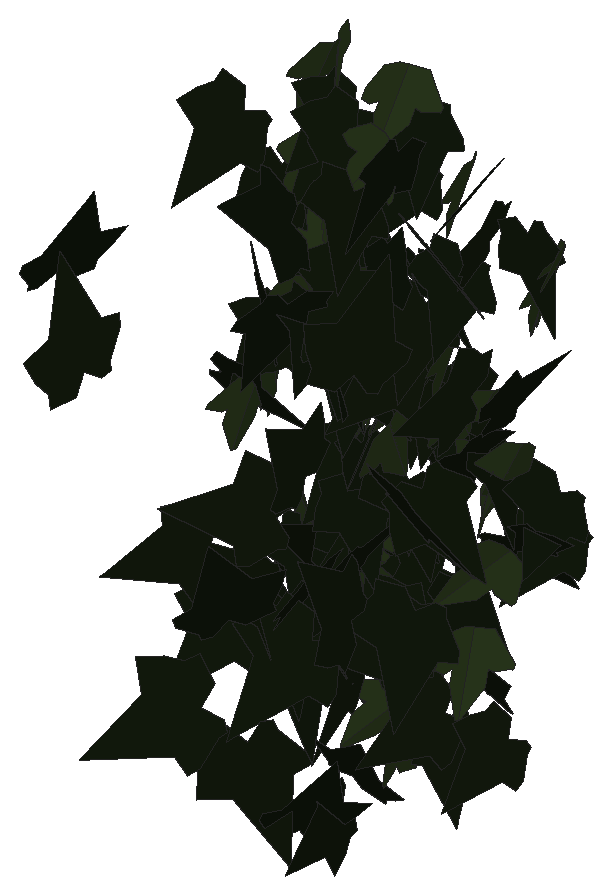
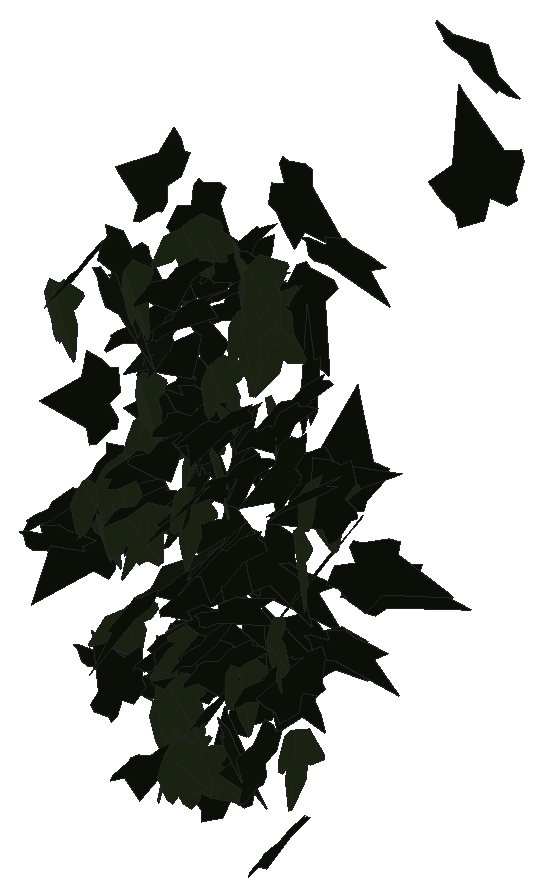
# SketchUp Ruby script. Lengths in inches.
U = 1.inch
M = Sketchup.active_model
def pt(a) = Geom::Point3d.new(a.map { |v| v * U })
def face(e, loops, mat)
  f = e.add_face(loops[0].map { |a| pt(a) })
  loops[1..].each { |l| e.add_face(l.map { |a| pt(a) }).erase! }
  f.material = f.back_material = mat if mat
  f
end
# faces: each face lists its corners as indices into pts; further lists are holes
def faces(e, pts, list, mat = nil) = list.each { |f| face(e, (f[0].is_a?(Array) ? f : [f]).map { |l| l.map { |i| pts[i] } }, mat) }
# xy, xz, yz: faces in a plane at the given z, y or x. An outline is a flat list of corners, or four numbers for a rectangle; further outlines are holes
def ring(l) = l.size == 4 ? [[l[0], l[1]], [l[2], l[1]], [l[2], l[3]], [l[0], l[3]]] : l.each_slice(2).to_a
def flat(e, list, mat, &to3) = list.each { |f| face(e, (f[0].is_a?(Array) ? f : [f]).map { |l| ring(l).map { |u, v| to3.(u, v) } }, mat) }
def xy(e, z, list, mat = nil) = flat(e, list, mat) { |x, y| [x, y, z] }
def xz(e, y, list, mat = nil) = flat(e, list, mat) { |x, z| [x, y, z] }
def yz(e, x, list, mat = nil) = flat(e, list, mat) { |y, z| [x, y, z] }
def lines(e, pts, list) = list.each { |a, b| e.add_line(pt(pts[a]), pt(pts[b])) }
# prism: a flat outline (further loops are holes) pulled along v
def prism(e, loops, v, mat = nil)
  f = face(e, loops, mat); d = Geom::Vector3d.new(v.map { |x| x * U })
  f.pushpull(f.normal.samedirection?(d) ? d.length : -d.length)
end
def box(e, o, s, mat = nil) = prism(e, [[o, [o[0] + s[0], o[1], o[2]], [o[0] + s[0], o[1] + s[1], o[2]], [o[0], o[1] + s[1], o[2]]]], [0, 0, s[2]], mat)
def at(x, y, z, deg = 0) = Geom::Transformation.translation(pt([x, y, z])) * Geom::Transformation.rotation(ORIGIN, Z_AXIS, deg.degrees)
def axes(o, x, y, z) = Geom::Transformation.new([*x, 0, *y, 0, *z, 0, *pt(o).to_a, 1])
def part(name) = M.definitions.add(name)
# library, detail: a bought-in or finely detailed component or shape, given as its bounding box
def library(name, o, s) = part(name).tap { |d| box(d.entities, o, s) }
def detail(e, o, s) = box(e.add_group.entities, o, s)
def put(e, d, t, mat = nil) = e.add_instance(d, t).tap { |i| i.material = mat if mat }
def group(e, t, mat = nil) = e.add_group.tap { |g| g.transformation = t; g.material = mat if mat }.entities
root = M.entities
M.materials.add("efeu1").color = [18, 25, 13]
M.materials.add("efeu2").color = [43, 57, 29]
c1 = part("ivyleaf_9")
p = [[1.54,2.16,1.25],[1.36,2.04,1.19],[-0.21,0.99,0.68],[-0.71,1.11,0.82],[-0.85,0.86,0.67],[-0.8,0.17,0.21],
  [-0.9,-0.01,0.1],[-0.67,-0.16,-0.02],[-0.08,-0.08,-0.05],[-0.03,-0.6,-0.4],[0.65,-0.88,-0.66],[0.83,-0.6,-0.49],
  [1.29,-0.42,-0.43],[1.8125,-0.07,-0.26],[1.21,0.44,0.15]]
faces(c1.entities,p,[[0,1,2,3,4,5,6,7,8,9,10,11,12,13,14]],"efeu1")
c2 = part("ivyleaf_10")
p = [[0,0.5,-0.03],[-0.0625,2.02,-0.43],[-0.19,2.01,-0.46],[-0.54,1.05,-0.29],[-0.52,0.625,-0.18],[-0.83,0.76,-0.28],
  [-1.16,0.64,-0.33],[-1.15,0.33,-0.24],[-0.77,-0.39,0.02],[-0.3,-0.51,0.16],[0.04,-0.48,0.23],[-0.02,2.01,-0.4375],
  [-0.06,2.01,-0.43],[0.04,-0.49,0.23],[0.67,-0.49,0.14],[1.38,0.36,-0.2],[1.375,0.51,-0.24],[0.81,0.65,-0.19],
  [0.62,0.59,-0.15],[0.6,1.09,-0.28],[0.5,1.23,-0.31]]
faces(c2.entities,p,[[0,1,2,3,4,5,6,7,8,9,10],[11,12,0,13,14,15,16,17,18,19,20]],"efeu2")
put(root,c1,axes([586.75,103.9375,300.07],[-1.43697,0.25356,-0.39672],[-0.40228,0.00084,1.45765],[0.24464,1.49073,0.06665]))
put(root,c1,axes([580.63,110.38,299],[0.80023,1.1061,0.65598],[-0.38497,-0.53115,1.36522],[1.22701,-0.88802,0.00051]))
put(root,c1,axes([584.13,113.52,281.39],[-1.16182,-0.52267,0.7875],[-0.71796,-0.32355,-1.27397],[0.61471,-1.36576,0.00044]))
put(root,c1,axes([585.37,113.77,285.38],[0.86867,0.58087,1.00057],[-0.81836,-0.57596,1.04485],[0.81783,-1.19332,-0.01725]))
put(root,c1,axes([589.24,113.0625,292.68],[-0.47842,0.80905,1.0484],[-0.56196,0.88534,-0.93966],[-1.19913,-0.7377,0.02208]))
put(root,c1,axes([585.23,115.08,279.55],[-0.59414,-0.71943,-1.18347],[0.79414,0.87809,-0.93247],[1.13469,-0.99125,0.03293]))
put(root,c1,axes([590.02,114.63,286.51],[-0.82384,0.13634,-1.1871],[-1.19412,-0.04146,0.82395],[0.04349,1.44437,0.1357]))
put(root,c1,axes([586.875,115.93,276.61],[0.99318,0.88272,0.41487],[-0.31395,-0.27126,1.32874],[0.92344,-1.0416,0.00555]))
put(root,c1,axes([587.57,117.14,276.97],[0.02429,-0.43729,-1.21261],[0.81544,-0.93412,0.35319],[-0.99836,-0.7736,0.25898]))
put(root,c1,axes([584.55,117.18,287.53],[-0.67759,-0.1305,1.15622],[-1.11265,-0.31875,-0.68804],[0.34039,-1.30168,0.05257]))
put(root,c1,axes([585.93,116.39,300.05],[-0.34419,0.20999,-1.38623],[-1.34021,-0.46852,0.26179],[-0.4118,1.34929,0.30664]))
put(root,c1,axes([585.91,117.46,282.89],[-1.34941,-0.66672,0.05597],[-0.05103,-0.02307,-1.50513],[0.66711,-1.35037,-0.00192]))
put(root,c1,axes([581.37,117.58,285.15],[-0.15915,-0.22662,-1.32348],[-0.57593,-1.19241,0.27343],[-1.21296,0.59591,0.04382]))
put(root,c1,axes([585.25,117.13,296.08],[-0.01644,1.00641,-0.92606],[0.05511,-0.92488,-1.00611],[-1.36653,-0.04941,-0.02943]))
put(root,c1,axes([588.62,116.69,295.01],[-0.73567,-0.51703,1.10661],[0.95074,0.5686,0.89771],[-0.7668,1.20103,0.05138]))
put(root,c1,axes([583.59,118.55,283.49],[0.59643,-1.16339,-0.67837],[0.3067,-0.60509,1.30737],[-1.31134,-0.67066,-0.00278]))
put(root,c1,axes([589.88,118.38,284.96],[-0.31241,-1.44345,0.12125],[0.04691,-0.13405,-1.47502],[1.44778,-0.30714,0.07396]))
put(root,c1,axes([585.31,118.65,294.98],[-0.05503,-1.06245,0.60991],[0.01412,-0.61103,-1.06314],[1.22499,-0.04068,0.03965]))
put(root,c1,axes([589.23,118.1,289.51],[1.02422,-0.74101,0.78859],[0.65085,-0.44562,-1.26405],[0.86451,1.21339,0.01737]))
put(root,c1,axes([585.54,118.18,284.93],[-0.65386,0.991,-0.59397],[0.25392,-0.54255,-1.18473],[-1.12712,-0.69712,0.07767]))
put(root,c1,axes([590.31,118.61,299.625],[0.69046,-0.84039,0.77859],[0.58148,-0.52618,-1.08361],[0.98709,0.89781,0.09373]))
put(root,c1,axes([581.75,118.77,282.01],[-1.28329,-0.42191,0.02426],[-0.0225,-0.00923,-1.35086],[0.42201,-1.28348,0.00174]))
put(root,c1,axes([591.98,118.76,294.17],[-1.15821,0.86921,0.23179],[-0.22706,0.08317,-1.44646],[-0.87046,-1.17824,0.06889]))
put(root,c1,axes([586.01,120.07,296.42],[-0.66991,-1.09414,0.35514],[-0.14803,-0.32555,-1.28224],[1.14076,-0.68478,0.04216]))
put(root,c1,axes([581.82,120.22,293.23],[-0.19244,0.08248,1.46618],[0.29567,-1.44626,0.12017],[1.43843,0.30831,0.17145]))
put(root,c1,axes([588.39,120.34,282.33],[-0.67766,-0.26939,1.09771],[-0.95641,-0.54541,-0.72428],[0.60235,-1.16907,0.08495]))
put(root,c1,axes([580.71,120.23,300.82],[-1.32776,-0.38705,-0.13705],[0.13425,0.02916,-1.38299],[0.38803,-1.33449,0.00953]))
put(root,c1,axes([585.42,120.58,299.11],[-0.10894,-1.25254,0.23472],[-0.01925,-0.23393,-1.25727],[1.2742,-0.11062,0.00108]))
put(root,c2,axes([584.23,119.79,295.39],[-1.08822,-0.53728,-0.16161],[0.13842,0.08466,-1.21354],[0.54372,-1.0969,-0.0145]))
put(root,c1,axes([589.26,119.76,289],[0.29444,-0.93222,-0.91034],[-0.03406,0.92747,-0.96078],[1.30253,0.23498,0.18066]))
put(root,c1,axes([585.85,119.1,284.73],[-0.18735,1.29671,-0.4513],[-0.06196,0.44704,1.31017],[1.3716,0.19731,-0.00246]))
put(root,c2,axes([584.5625,119.88,296.85],[0.00626,1.18118,-0.33334],[-0.04412,0.33335,1.18037],[1.22652,0.00597,0.04416]))
put(root,c2,axes([580.87,120.67,289.8],[-0.24847,-1.19559,0.25512],[-0.03544,-0.25318,-1.22103],[1.22199,-0.25044,0.01646]))
put(root,c1,axes([588.68,121.39,279.3],[-0.76134,-0.69541,0.66115],[-0.51321,-0.418,-1.03066],[0.81076,-0.91762,-0.03155]))
put(root,c1,axes([586.87,121.15,300.88],[-0.31952,0.5689,-1.11645],[0.58698,-0.94999,-0.65207],[-1.10706,-0.6679,-0.0235]))
put(root,c2,axes([587.12,120.54,290.31],[-0.03534,-1.14369,-0.54348],[0.12274,0.53804,-1.14022],[1.26029,-0.08447,0.09581]))
put(root,c1,axes([579.8,120.64,290],[1.09104,-0.14552,0.48254],[0.47176,-0.11007,-1.09987],[0.17737,1.1879,-0.0428]))
put(root,c1,axes([591.54,121.36,279.26],[-1.1233,-0.29497,-0.01693],[0.01529,0.00843,-1.16137],[0.29506,-1.12339,-0.00427]))
put(root,c1,axes([586.87,121.52,292.49],[-1.23494,-0.25607,0.11644],[-0.11429,-0.02234,-1.26121],[0.25703,-1.24022,-0.00133]))
put(root,c1,axes([581.96,121.41,281.42],[-0.83171,-0.34084,-1.08607],[1.02621,0.35752,-0.89807],[0.49256,-1.3204,0.03718]))
put(root,c1,axes([583.74,122.02,291.15],[0.66105,-0.38263,-1.12476],[1.04165,-0.43235,0.75929],[-0.57136,-1.23091,0.08294]))
put(root,c1,axes([586.2,121.57,291.09],[-0.76954,0.54326,-0.84018],[0.6935,-0.47439,-0.94193],[-0.72117,-1.03588,-0.00926]))
put(root,c1,axes([584.57,121.67,275.34],[1.22856,-0.19127,-0.04988],[0.05042,-0.00036,1.24333],[-0.19113,-1.22957,0.00739]))
put(root,c1,axes([587.27,122.15,294.65],[-0.39558,-1.15691,0.0657],[-0.01698,-0.06363,-1.22266],[1.15865,-0.39592,0.00452]))
put(root,c2,axes([590.68,121.88,285.8],[0.46461,0.67833,-0.96279],[-0.91103,-0.44894,-0.75593],[-0.74641,0.97019,0.32336]))
put(root,c2,axes([587.01,121.09,278.02],[0.30916,-0.96914,-0.74002],[0.06226,0.77498,-0.98891],[1.21777,0.20641,0.23843]))
put(root,c1,axes([586.54,122.1,281.55],[-1.0834,-0.07843,0.84395],[-0.84228,-0.05332,-1.08621],[0.09464,-1.37228,-0.00603]))
put(root,c1,axes([584.57,121.86,286.4375],[-0.00276,-1.11264,-0.44385],[-0.0281,0.44379,-1.11231],[1.19757,0.00785,-0.02713]))
put(root,c1,axes([584.58,121.41,292.02],[0.6626,-0.83511,-0.79781],[-0.29718,0.76553,-1.04814],[1.11606,0.69964,0.19456]))
put(root,c2,axes([585.59,121.82,300.3],[0.99735,-0.34559,-0.64031],[-0.6193,0.16712,-1.05484],[0.38196,1.17336,-0.03835]))
put(root,c1,axes([586.6875,121.09,295.23],[-0.13898,0.19601,1.4464],[-0.68699,1.27316,-0.23855],[-1.28784,-0.70032,-0.02884]))
put(root,c2,axes([589.45,122.14,281.95],[0.48686,1.1013,-0.37433],[-0.13705,-0.34865,-1.20402],[-1.15508,0.50556,-0.01492]))
put(root,c2,axes([581.07,121.89,278.92],[0.01123,-1.16228,-0.38586],[0.06741,0.38588,-1.16037],[1.22279,-0.0106,0.06751]))
put(root,c2,axes([581.67,122.96,298.38],[-0.07127,-0.80874,0.97025],[0.415,-0.93284,-0.74707],[1.19299,0.27619,0.31784]))
put(root,c2,axes([584.9,122.24,290.69],[0.8024,-0.86614,-0.24766],[-0.14746,0.2009,-1.18037],[0.8887,0.81537,0.02776]))
put(root,c1,axes([583.64,122.83,300.19],[-1.05981,-0.61772,0.08652],[-0.07959,-0.03525,-1.22665],[0.61865,-1.06275,-0.0096]))
put(root,c2,axes([584.48,122.62,294.61],[0.08564,-1.18686,0.26369],[-0.00831,-0.26491,-1.18965],[1.21578,0.0818,-0.0267]))
put(root,c1,axes([580.21,123.29,290.8125],[-0.60864,-0.84756,0.59812],[-0.03404,-0.67677,-0.99367],[1.0368,-0.51978,0.31849]))
put(root,c1,axes([588.18,123.16,296.02],[-0.32572,-1.17556,0.2203],[-0.0433,-0.21659,-1.21975],[1.19524,-0.32821,0.01585]))
put(root,c1,axes([580.19,122.79,282.2],[1.22783,0.05822,-0.30725],[0.29319,0.21859,1.2131],[0.10875,-1.24667,0.19835]))
put(root,c1,axes([583.6875,122.96,278.64],[-1.02816,0.37299,-0.69527],[0.64215,-0.26797,-1.09337],[-0.45843,-1.2119,0.02778]))
put(root,c1,axes([583.38,123.25,290.88],[-0.2472,-1.22327,-0.03463],[0.00337,0.03465,-1.24799],[1.22376,-0.2472,-0.00356]))
put(root,c1,axes([586.74,122.8,295.8125],[0.87876,-0.86198,0.0072],[0.01438,0.00437,-1.23088],[0.86189,0.87878,0.01319]))
put(root,c2,axes([587.85,122.96,293.01],[0.40098,-1.14063,0.09568],[0.00698,-0.09894,-1.20878],[1.14462,0.40019,-0.02615]))
put(root,c2,axes([581.68,122.7,294.08],[0.59049,-0.97092,-0.40967],[-0.16058,0.38122,-1.13494],[1.0415,0.60925,0.05728]))
put(root,c1,axes([581.27,123.65,282.6],[-0.21022,-1.21149,0.13054],[-0.02307,-0.12849,-1.22959],[1.21828,-0.21148,-0.00075]))
put(root,c1,axes([582.61,123.99,300.01],[-0.7286,-0.83948,0.60918],[-0.0813,-0.69595,-1.05628],[1.03403,-0.64624,0.3462]))
put(root,c1,axes([585.125,123.39,293.03],[-0.40797,-1.06567,-0.40812],[0.10426,0.3968,-1.14033],[1.13637,-0.419,-0.0419]))
put(root,c2,axes([587.29,122.75,278.82],[-0.33338,0.2022,1.11857],[-1.11015,0.19256,-0.36567],[-0.24425,-1.1512,0.1353]))
put(root,c2,axes([584.78,123.72,277.37],[-0.39835,-0.58287,0.93557],[-0.40614,-0.8472,-0.70074],[1.02474,-0.56236,0.08597]))
put(root,c1,axes([583.9,123.16,287.45],[0.58523,-0.97766,-0.35902],[-0.06212,0.37831,-1.13147],[1.03964,0.57295,0.13449]))
put(root,c2,axes([588.14,122.78,290.93],[0.05039,-1.07273,-0.61116],[0.116,0.61307,-1.06653],[1.22915,-0.01388,0.12571]))
put(root,c1,axes([585.28,123.88,286.17],[0.10591,-1.3936,0.29794],[0.48399,-0.24583,-1.3219],[1.34039,0.19888,0.45377]))
put(root,c1,axes([588.66,122.55,289.14],[0.19053,1.21252,0.02993],[0.00031,0.03025,-1.22739],[-1.21289,0.19048,0.00439]))
put(root,c1,axes([590.32,122.32,291.37],[0.40517,0.16812,1.16004],[0.61177,1.01662,-0.36101],[-0.99984,0.69016,0.2492]))
put(root,c1,axes([584.48,123.87,284.24],[-1.04754,-0.44709,0.3561],[-0.33218,-0.12882,-1.13891],[0.46514,-1.09889,-0.01137]))
put(root,c1,axes([586.6875,123.95,291.07],[-0.35355,-1.14373,0.02371],[-0.00755,-0.02248,-1.19712],[1.14395,-0.35363,-0.00057]))
put(root,c1,axes([586.95,123.7,277.15],[-0.11616,-1.1363,-0.36793],[0.08005,0.36143,-1.14149],[1.1917,-0.13504,0.04082]))
put(root,c1,axes([590.66,123.75,297.86],[0.43853,-1.1551,-0.0698],[-0.0257,0.0649,-1.23554],[1.15692,0.43928,-0.00099]))
put(root,c1,axes([588.01,123.13,283.54],[0.64097,-0.8595,-0.77315],[-0.3532,0.69617,-1.06674],[1.10079,0.72384,0.10792]))
put(root,c2,axes([582.5625,123.54,282.29],[0.04546,-1.20316,-0.00895],[-0.00173,0.00889,-1.20402],[1.20319,0.04547,-0.00139]))
put(root,c1,axes([588.23,124,279.6],[0.02208,-0.4541,1.10739],[0.74425,-0.8622,-0.3684],[0.93734,0.69528,0.26642]))
put(root,c1,axes([584.67,123.9375,281.52],[0.70743,0.18214,1.06469],[-1.02408,-0.29165,0.73034],[0.34351,-1.24457,-0.01534]))
put(root,c1,axes([589.27,123.21,297.45],[-0.81048,0.97289,0.13476],[-0.07226,0.11517,-1.26612],[-0.97952,-0.81349,-0.01809]))
put(root,c1,axes([588.62,122.84,299.01],[-0.23622,1.2174,0.3214],[-0.0803,0.31177,-1.23996],[-1.25655,-0.24879,0.01882]))
put(root,c2,axes([579.65,123.53,289.13],[0.57346,-1.06817,-0.28581],[-0.06016,0.29134,-1.20956],[1.10411,0.57067,0.08254]))
put(root,c1,axes([581.14,123.91,278.99],[0.80786,-0.80528,0.41415],[0.2853,-0.3004,-1.14061],[0.85942,0.85669,-0.01066]))
put(root,c1,axes([588.82,124.22,288.13],[0.3666,-1.08139,0.36484],[0.1634,-0.32952,-1.14089],[1.12952,0.39865,0.04663]))
put(root,c1,axes([585.99,124.63,282.67],[-0.51878,-0.74615,0.8101],[-0.34182,-0.74218,-0.90248],[1.04698,-0.61203,0.10676]))
put(root,c1,axes([584.68,124.13,289.43],[0.75073,-0.93582,0.37261],[0.21011,-0.309,-1.1994],[0.98511,0.77907,-0.02814]))
put(root,c1,axes([584.91,124.7,298.13],[-0.47105,-0.99751,0.48523],[-0.1023,-0.48585,-1.09811],[1.10454,-0.47041,0.10523]))
put(root,c2,axes([581.2,123.125,283.97],[-0.06314,0.0881,-1.26129],[-0.7809,0.99049,0.10827],[0.99439,0.78343,0.00494]))
put(root,c1,axes([590.25,123.22,286.02],[1.15034,0.58383,0.06138],[0.04391,0.04908,-1.28979],[-0.5854,1.15093,0.02386]))
put(root,c1,axes([591.18,124.73,287.37],[-0.35974,-1.08939,0.37573],[-0.02624,-0.38577,-1.14361],[1.15206,-0.34896,0.09128]))
put(root,c2,axes([584.69,123.38,283.11],[-0.45837,-0.53801,-0.98206],[0.68844,0.70151,-0.70564],[0.88314,-0.82609,0.04036]))
put(root,c2,axes([589.41,124.45,288.42],[-0.13218,-1.08736,0.51445],[-0.05423,-0.51163,-1.09534],[1.20169,-0.14269,0.00715]))
put(root,c1,axes([579.23,124.41,296.3],[0.05504,-1.22935,-0.15101],[-0.01352,0.15056,-1.23056],[1.23852,0.05627,-0.00672]))
put(root,c2,axes([591.14,124.2,296.38],[0.33834,-1.17623,0.08488],[0.01108,-0.08513,-1.22386],[1.17924,0.33828,-0.01285]))
put(root,c2,axes([584.73,124.24,301.74],[0.58458,0.97134,-0.52329],[-0.35337,-0.39618,-1.13015],[-1.04521,0.6772,0.08942]))
put(root,c1,axes([583.72,124.59,283.75],[0.01057,-1.17001,0.11036],[0.02015,-0.11017,-1.16991],[1.17504,0.01241,0.01907]))
put(root,c2,axes([585.87,123.78,278.05],[-0.68941,0.91652,0.1856],[-0.12115,0.1411,-1.1468],[-0.92724,-0.69987,0.01184]))
put(root,c1,axes([582.72,124.64,283.37],[-0.2241,-1.20586,-0.16397],[0.02242,0.16261,-1.22648],[1.21675,-0.22509,-0.0076]))
put(root,c1,axes([580.14,124.76,294.99],[-0.23403,-1.20485,0.00017],[-0.00041,-0.0001,-1.22737],[1.20485,-0.23403,-0.00039]))
put(root,c2,axes([588.61,124.59,287.65],[0.62149,-1.0098,0.3924],[0.191,-0.34316,-1.18562],[1.06639,0.64997,-0.01633]))
put(root,c1,axes([591.44,124.74,286.06],[-1.04845,-0.50566,0.05649],[-0.03124,-0.06516,-1.16315],[0.50785,-1.04795,0.04507]))
put(root,c1,axes([582.36,125,285.96],[-0.81315,-0.82316,0.29498],[-0.09613,-0.31623,-1.14743],[0.86912,-0.80513,0.14908]))
put(root,c2,axes([584.71,124.89,278.1875],[-0.19608,-0.82391,0.82247],[-0.01525,-0.83217,-0.83726],[1.16407,-0.14969,0.12757]))
put(root,c1,axes([582.93,124.65,281.45],[0.28235,-1.1379,0.02621],[0.00586,-0.02555,-1.17241],[1.13819,0.28241,-0.00047]))
put(root,c2,axes([584.79,124.1,289.49],[0.01561,-1.19293,-0.36658],[-0.03663,0.36602,-1.19264],[1.24745,0.02568,-0.03043]))
put(root,c1,axes([587.11,123.93,290.61],[0.38511,-0.79395,-0.89057],[-0.1156,0.90658,-0.85821],[1.18748,0.34574,0.20527]))
put(root,c2,axes([580.89,124.72,301.24],[0.05681,-1.18756,0.38494],[-0.03141,-0.38657,-1.18797],[1.24799,0.04433,-0.04742]))
put(root,c2,axes([587.95,124.74,289.875],[-0.13398,-1.11855,0.43094],[-0.00869,-0.4327,-1.12583],[1.19866,-0.12816,0.04]))
put(root,c2,axes([587.18,124.64,298.81],[0.4266,-1.13929,0.21512],[0.06123,-0.20676,-1.21645],[1.15781,0.43071,-0.01493]))
put(root,c1,axes([586.72,124.93,289.09],[-0.25581,-1.17212,-0.08039],[0.01176,0.07971,-1.1997],[1.17482,-0.25602,-0.0055]))
put(root,c1,axes([579.59,124.86,276.38],[0.25066,-1.1436,0.04901],[0.00402,-0.04929,-1.17073],[1.14465,0.2506,-0.00662]))
put(root,c2,axes([591.07,124.75,296.64],[0.63363,-1.03128,0.22207],[0.08222,-0.20999,-1.20975],[1.05171,0.63774,-0.03922]))
put(root,c1,axes([584.52,125.15,289.56],[0.02203,-1.17693,0.31025],[0.08442,-0.30808,-1.17468],[1.21421,0.04277,0.07605]))
put(root,c1,axes([579.2,124.46,293.2],[1.03015,-0.62215,0.06083],[0.05586,-0.02518,-1.20343],[0.62262,1.03164,0.00732]))
put(root,c2,axes([586.48,125.02,287.83],[-0.05944,0.88199,-0.84663],[-0.02779,-0.84839,-0.88187],[-1.22226,-0.02361,0.06123]))
put(root,c2,axes([587.02,125.05,288.36],[-0.66247,-0.72618,0.68666],[-0.20502,-0.70755,-0.94607],[0.97817,-0.64011,0.26675]))
put(root,c2,axes([581.2,125.24,301.46],[-0.40385,0.31003,-1.11864],[0.36644,-1.0898,-0.43433],[-1.10145,-0.47623,0.26566]))
put(root,c2,axes([581.55,124.69,298.84],[0.10989,-1.23376,0.036],[0.00514,-0.03569,-1.23864],[1.23427,0.10999,0.00195]))
put(root,c1,axes([582.81,124.72,294.12],[0.12612,-1.12315,-0.43539],[0.09156,0.44544,-1.12256],[1.2011,0.08398,0.13129]))
put(root,c1,axes([584.92,125.14,300.07],[-0.1679,-1.22182,-0.05686],[0.00696,0.05644,-1.23331],[1.22313,-0.16805,-0.00079]))
put(root,c2,axes([584.55,125.11,281.28],[-0.09576,-1.11654,0.51532],[-0.03417,-0.51427,-1.1206],[1.22925,-0.10127,0.00899]))
